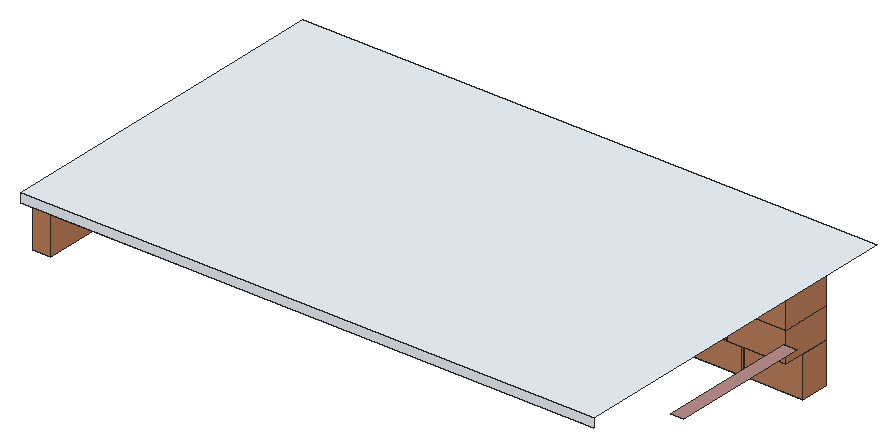
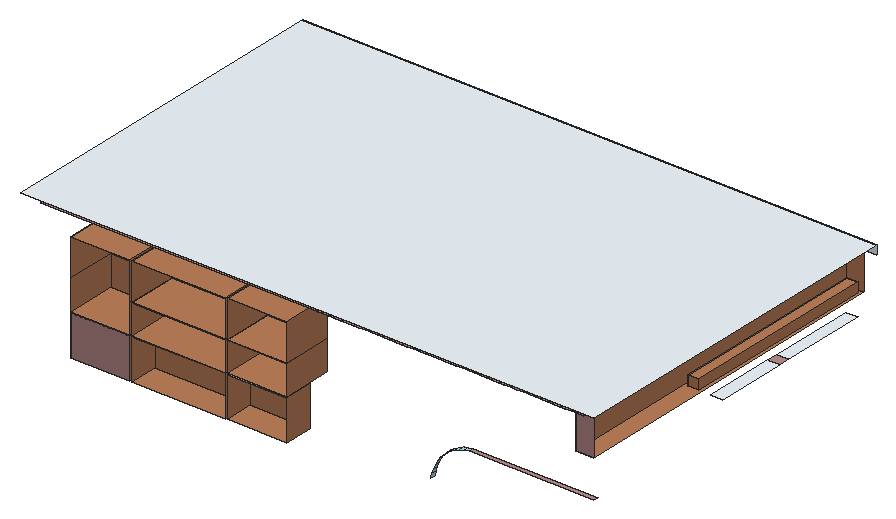
# SketchUp Ruby script. Lengths in inches.
U = 1.inch
M = Sketchup.active_model
def pt(a) = Geom::Point3d.new(a.map { |v| v * U })
def face(e, loops, mat)
  f = e.add_face(loops[0].map { |a| pt(a) })
  loops[1..].each { |l| e.add_face(l.map { |a| pt(a) }).erase! }
  f.material = f.back_material = mat if mat
  f
end
# faces: each face lists its corners as indices into pts; further lists are holes
def faces(e, pts, list, mat = nil) = list.each { |f| face(e, (f[0].is_a?(Array) ? f : [f]).map { |l| l.map { |i| pts[i] } }, mat) }
# xy, xz, yz: faces in a plane at the given z, y or x. An outline is a flat list of corners, or four numbers for a rectangle; further outlines are holes
def ring(l) = l.size == 4 ? [[l[0], l[1]], [l[2], l[1]], [l[2], l[3]], [l[0], l[3]]] : l.each_slice(2).to_a
def flat(e, list, mat, &to3) = list.each { |f| face(e, (f[0].is_a?(Array) ? f : [f]).map { |l| ring(l).map { |u, v| to3.(u, v) } }, mat) }
def xy(e, z, list, mat = nil) = flat(e, list, mat) { |x, y| [x, y, z] }
def xz(e, y, list, mat = nil) = flat(e, list, mat) { |x, z| [x, y, z] }
def yz(e, x, list, mat = nil) = flat(e, list, mat) { |y, z| [x, y, z] }
def lines(e, pts, list) = list.each { |a, b| e.add_line(pt(pts[a]), pt(pts[b])) }
# prism: a flat outline (further loops are holes) pulled along v
def prism(e, loops, v, mat = nil)
  f = face(e, loops, mat); d = Geom::Vector3d.new(v.map { |x| x * U })
  f.pushpull(f.normal.samedirection?(d) ? d.length : -d.length)
end
def box(e, o, s, mat = nil) = prism(e, [[o, [o[0] + s[0], o[1], o[2]], [o[0] + s[0], o[1] + s[1], o[2]], [o[0], o[1] + s[1], o[2]]]], [0, 0, s[2]], mat)
def at(x, y, z, deg = 0) = Geom::Transformation.translation(pt([x, y, z])) * Geom::Transformation.rotation(ORIGIN, Z_AXIS, deg.degrees)
def axes(o, x, y, z) = Geom::Transformation.new([*x, 0, *y, 0, *z, 0, *pt(o).to_a, 1])
def part(name) = M.definitions.add(name)
# library, detail: a bought-in or finely detailed component or shape, given as its bounding box
def library(name, o, s) = part(name).tap { |d| box(d.entities, o, s) }
def detail(e, o, s) = box(e.add_group.entities, o, s)
def put(e, d, t, mat = nil) = e.add_instance(d, t).tap { |i| i.material = mat if mat }
def group(e, t, mat = nil) = e.add_group.tap { |g| g.transformation = t; g.material = mat if mat }.entities
root = M.entities
M.materials.add("[0093_AliceBlue]").color = [240, 248, 255]
M.materials.add("[0095_LightBlue]").color = [173, 216, 230]
M.materials.add("[0119_RosyBrown]").color = [188, 143, 143]
M.materials.add("[Wood Veneer 02]").color = [190, 128, 91]
c1 = library("Group\#6",[-0.5,-0.5,0],[175.45,81.95,0.375])
xy(root,86.86,[[126.39,126.49,150.39,137.93],[151.09,126.49,188.68,137.93],[189.375,126.49,213.375,137.93]],"[Wood Veneer 02]")
xy(root,102.8,[[126.39,126.49,150.39,137.93]],"[0119_RosyBrown]")
xy(root,103.11,[[151.09,126.49,188.68,137.93],[189.375,126.49,213.375,137.93]],"[0119_RosyBrown]")
xy(root,103.42,[[126.39,117.86,150.39,137.93],[151.09,117.86,188.68,137.93],[189.375,117.86,213.375,137.93]],"[Wood Veneer 02]")
xy(root,107.93,[[4.97,133.77,55.03,135.55]],"[0119_RosyBrown]")
xy(root,115.3,[[126.39,117.86,150.39,137.93],[151.09,117.86,188.68,137.93]],"[Wood Veneer 02]")
xy(root,115.49,[[126.39,117.86,150.39,137.93],[151.09,117.86,188.68,137.93]],"[Wood Veneer 02]")
xy(root,119.86,[[0,9.26,4.95,43.72],[0,48.29,4.95,77.05]],"[0093_AliceBlue]")
xy(root,119.86,[[0,43.72,4.95,48.29]],"[0119_RosyBrown]")
xy(root,121.64,[[225.375,45.11,230.5,101.93]],"[0119_RosyBrown]")
xy(root,123.05,[[[4.95,0,12.13,135.55],[6.31,1.36,10.77,81.01]]],"[Wood Veneer 02]")
xy(root,126.8,[[6.31,1.36,10.77,81.01]],"[Wood Veneer 02]")
xy(root,130.36,[[126.39,117.86,150.39,137.93],[151.09,117.86,188.68,137.93],[189.375,117.86,213.375,137.93]],"[Wood Veneer 02]")
xy(root,138.36,[[12.13,0,225.125,5.1875],[12.13,5.1875,12.13,12.37,217.95,12.37,217.95,124.69,12.13,124.69,12.13,131.86,225.125,131.86,225.125,5.1875],[[12.13,12.37,217.95,124.69],[37.92,26.16,192.16,26.16,193.72,26.26,195.26,26.56,196.75,27.07,198.16,27.76,199.46,28.64,200.64,29.67,201.68,30.85,202.55,32.16,203.24,33.5625,203.75,35.05,204.05,36.59,204.16,38.16,204.16,98.89,204.05,100.46,203.75,102,203.24,103.49,202.55,104.89,201.68,106.2,200.64,107.38,199.46,108.42,198.16,109.29,196.75,109.98,195.26,110.49,193.72,110.79,192.16,110.89,37.92,110.89,36.35,110.79,34.8125,110.49,33.33,109.98,31.92,109.29,30.61,108.42,29.43,107.38,28.4,106.2,27.53,104.89,26.83,103.49,26.33,102,26.02,100.46,25.92,98.89,25.92,38.16,26.16,36.65,26.58,35.18,27.16,33.76,27.9,32.42,28.78,31.17,29.8,30.03,30.9375,29.02,32.18,28.13,33.52,27.4,34.9375,26.82,36.41,26.4]],[[38.07,28.05,36.82,28.26,35.56,28.61,34.34,29.11,33.19,29.74,32.12,30.5,31.14,31.375,30.26,32.36,29.51,33.43,28.87,34.58,28.375,35.8,28.02,37.06,27.8125,38.31,27.8125,98.89,27.9,100.21,28.16,101.51,28.58,102.76,29.17,103.95,29.9,105.05,30.77,106.04,31.77,106.91,32.87,107.65,34.05,108.23,35.3,108.66,36.6,108.91,37.92,109,192.16,109,193.48,108.91,194.77,108.66,196.02,108.23,197.21,107.65,198.31,106.91,199.3,106.04,200.17,105.05,200.91,103.95,201.49,102.76,201.92,101.51,202.18,100.21,202.26,98.89,202.26,38.16,202.18,36.84,201.92,35.54,201.49,34.29,200.91,33.1,200.17,32,199.3,31.01,198.31,30.14,197.21,29.4,196.02,28.82,194.77,28.4,193.48,28.14,192.16,28.05],[49.92,38.16,180.16,38.16,181.72,38.26,183.26,38.56,184.75,39.07,186.16,39.76,187.46,40.64,188.64,41.67,189.68,42.85,190.55,44.16,191.24,45.5625,191.75,47.05,192.05,48.59,192.16,50.16,192.16,86.89,192.05,88.46,191.75,90,191.24,91.49,190.55,92.89,189.68,94.2,188.64,95.38,187.46,96.42,186.16,97.29,184.75,97.98,183.26,98.49,181.72,98.79,180.16,98.89,49.92,98.89,48.35,98.79,46.8125,98.49,45.33,97.98,43.92,97.29,42.61,96.42,41.43,95.38,40.4,94.2,39.53,92.89,38.83,91.49,38.33,90,38.02,88.46,37.92,86.89,37.92,50.16,37.97,48.57,38.24,47.01,38.72,45.5,39.4,44.07,40.27,42.74,41.31,41.55,42.5,40.51,43.83,39.64,45.26,38.96,46.77,38.48,48.33,38.21]],[49.83,40.68,48.59,40.72,47.37,40.93,46.1875,41.31,45.07,41.84,44.03,42.52,43.1,43.34,42.28,44.27,41.6,45.31,41.07,46.43,40.7,47.61,40.49,48.83,40.44,50.07,40.44,86.89,40.53,88.13,40.77,89.35,41.17,90.52,41.71,91.63,42.4,92.66,43.22,93.59,44.15,94.41,45.18,95.1,46.29,95.65,47.47,96.04,48.68,96.29,49.92,96.37,180.16,96.37,181.39,96.29,182.61,96.04,183.78,95.65,184.89,95.1,185.92,94.41,186.85,93.59,187.67,92.66,188.36,91.63,188.91,90.52,189.31,89.35,189.55,88.13,189.63,86.89,189.63,50.16,189.55,48.92,189.31,47.7,188.91,46.53,188.36,45.42,187.67,44.39,186.85,43.46,185.92,42.64,184.89,41.95,183.78,41.4,182.61,41.01,181.39,40.76,180.16,40.68]],"[0093_AliceBlue]")
xy(root,138.36,[[225.125,0,225.125,131.86,12.13,131.86,12.13,135.55,11.89,135.55,11.89,137.93,14.71,137.93,14.71,135.55,16.77,135.55,16.77,137.93,19.59,137.93,19.59,135.55,21.65,135.55,21.65,137.93,24.47,137.93,24.47,135.55,26.53,135.55,26.53,137.93,29.35,137.93,29.35,135.55,31.42,135.55,31.42,137.93,34.23,137.93,34.23,135.55,36.3,135.55,36.3,137.93,39.11,137.93,39.11,135.55,41.18,135.55,41.18,137.93,43.99,137.93,43.99,135.55,46.06,135.55,46.06,137.93,48.875,137.93,48.875,135.55,50.9375,135.55,50.9375,137.93,53.76,137.93,53.76,135.55,55.82,135.55,55.82,137.93,58.64,137.93,58.64,135.55,60.7,135.55,60.7,137.93,63.52,137.93,63.52,135.55,65.58,135.55,65.58,137.93,68.4,137.93,68.4,135.55,70.46,135.55,70.46,137.93,73.28,137.93,73.28,135.55,75.34,135.55,75.34,137.93,78.16,137.93,78.16,135.55,80.22,135.55,80.22,137.93,83.04,137.93,83.04,135.55,85.1,135.55,85.1,137.93,87.92,137.93,87.92,135.55,89.98,135.55,89.98,137.93,92.8,137.93,92.8,135.55,94.86,135.55,94.86,137.93,97.68,137.93,97.68,135.55,99.74,135.55,99.74,137.93,102.5625,137.93,102.5625,135.55,104.625,135.55,104.625,137.93,107.44,137.93,107.44,135.55,109.51,135.55,109.51,137.93,112.32,137.93,112.32,135.55,114.39,135.55,114.39,137.93,225.375,137.93,225.375,0],[7.01,135.55,9.83,137.93],[9.83,135.55,11.89,137.93],[14.71,135.55,16.77,137.93],[19.59,135.55,21.65,137.93],
  [24.47,135.55,26.53,137.93],[29.35,135.55,31.42,137.93],[34.23,135.55,36.3,137.93],[39.11,135.55,41.18,137.93],[43.99,135.55,46.06,137.93],
  [48.875,135.55,50.9375,137.93],[53.76,135.55,55.82,137.93],[58.64,135.55,60.7,137.93],[63.52,135.55,65.58,137.93],[68.4,135.55,70.46,137.93],
  [73.28,135.55,75.34,137.93],[78.16,135.55,80.22,137.93],[83.04,135.55,85.1,137.93],[87.92,135.55,89.98,137.93],[92.8,135.55,94.86,137.93],
  [97.68,135.55,99.74,137.93],[102.5625,135.55,104.625,137.93],[107.44,135.55,109.51,137.93],[112.32,135.55,114.05,137.93],[114.05,135.55,114.39,137.93]],"[0119_RosyBrown]")
xy(root,138.92,[[[37.92,26.16,36.41,26.4,34.9375,26.82,33.52,27.4,32.18,28.13,30.9375,29.02,29.8,30.03,28.78,31.17,27.9,32.42,27.16,33.76,26.58,35.18,26.16,36.65,25.92,38.16,25.92,98.89,26.02,100.46,26.33,102,26.83,103.49,27.53,104.89,28.4,106.2,29.43,107.38,30.61,108.42,31.92,109.29,33.33,109.98,34.8125,110.49,36.35,110.79,37.92,110.89,192.16,110.89,193.72,110.79,195.26,110.49,196.75,109.98,198.16,109.29,199.46,108.42,200.64,107.38,201.68,106.2,202.55,104.89,203.24,103.49,203.75,102,204.05,100.46,204.16,98.89,204.16,38.16,204.05,36.59,203.75,35.05,203.24,33.5625,202.55,32.16,201.68,30.85,200.64,29.67,199.46,28.64,198.16,27.76,196.75,27.07,195.26,26.56,193.72,26.26,192.16,26.16],[38.07,28.05,192.16,28.05,193.48,28.14,194.77,28.4,196.02,28.82,197.21,29.4,198.31,30.14,199.3,31.01,200.17,32,200.91,33.1,201.49,34.29,201.92,35.54,202.18,36.84,202.26,38.16,202.26,98.89,202.18,100.21,201.92,101.51,201.49,102.76,200.91,103.95,200.17,105.05,199.3,106.04,198.31,106.91,197.21,107.65,196.02,108.23,194.77,108.66,193.48,108.91,192.16,109,37.92,109,36.6,108.91,35.3,108.66,34.05,108.23,32.87,107.65,31.77,106.91,30.77,106.04,29.9,105.05,29.17,103.95,28.58,102.76,28.16,101.51,27.9,100.21,27.8125,98.89,27.8125,38.31,28.02,37.06,28.375,35.8,28.87,34.58,29.51,33.43,30.26,32.36,31.14,31.375,32.12,30.5,33.19,29.74,34.34,29.11,35.56,28.61,36.82,28.26]]],"[0119_RosyBrown]")
xy(root,139.11,[[[49.92,38.16,48.33,38.21,46.77,38.48,45.26,38.96,43.83,39.64,42.5,40.51,41.31,41.55,40.27,42.74,39.4,44.07,38.72,45.5,38.24,47.01,37.97,48.57,37.92,50.16,37.92,86.89,38.02,88.46,38.33,90,38.83,91.49,39.53,92.89,40.4,94.2,41.43,95.38,42.61,96.42,43.92,97.29,45.33,97.98,46.8125,98.49,48.35,98.79,49.92,98.89,180.16,98.89,181.72,98.79,183.26,98.49,184.75,97.98,186.16,97.29,187.46,96.42,188.64,95.38,189.68,94.2,190.55,92.89,191.24,91.49,191.75,90,192.05,88.46,192.16,86.89,192.16,50.16,192.05,48.59,191.75,47.05,191.24,45.5625,190.55,44.16,189.68,42.85,188.64,41.67,187.46,40.64,186.16,39.76,184.75,39.07,183.26,38.56,181.72,38.26,180.16,38.16],[49.83,40.68,180.16,40.68,181.39,40.76,182.61,41.01,183.78,41.4,184.89,41.95,185.92,42.64,186.85,43.46,187.67,44.39,188.36,45.42,188.91,46.53,189.31,47.7,189.55,48.92,189.63,50.16,189.63,86.89,189.55,88.13,189.31,89.35,188.91,90.52,188.36,91.63,187.67,92.66,186.85,93.59,185.92,94.41,184.89,95.1,183.78,95.65,182.61,96.04,181.39,96.29,180.16,96.37,49.92,96.37,48.68,96.29,47.47,96.04,46.29,95.65,45.18,95.1,44.15,94.41,43.22,93.59,42.4,92.66,41.71,91.63,41.17,90.52,40.77,89.35,40.53,88.13,40.44,86.89,40.44,50.07,40.49,48.83,40.7,47.61,41.07,46.43,41.6,45.31,42.28,44.27,43.1,43.34,44.03,42.52,45.07,41.84,46.1875,41.31,47.37,40.93,48.59,40.72]]],"[0119_RosyBrown]")
xy(root,141.75,[[0,0,230.5,141.75]],"[0093_AliceBlue]")
xz(root,0,[[0,138.36,230.5,141.75]],"[0093_AliceBlue]")
xz(root,0,[[4.95,123.05,12.13,138.36]],"[Wood Veneer 02]")
xz(root,1.36,[[6.31,123.05,10.77,126.8]],"[Wood Veneer 02]")
xz(root,26.16,[[37.92,138.36,192.16,138.92]],"[0119_RosyBrown]")
xz(root,28.05,[[38.07,138.74,192.16,138.92]],"[0119_RosyBrown]")
xz(root,38.16,[[49.92,138.36,180.16,139.11]],"[0119_RosyBrown]")
xz(root,40.68,[[49.83,138.74,180.16,139.11]],"[0119_RosyBrown]")
xz(root,81.01,[[6.31,123.05,10.77,126.8]],"[Wood Veneer 02]")
xz(root,96.37,[[49.92,138.74,180.16,139.11]],"[0119_RosyBrown]")
xz(root,98.89,[[49.92,138.36,180.16,139.11]],"[0119_RosyBrown]")
xz(root,109,[[37.92,138.74,192.16,138.92]],"[0119_RosyBrown]")
xz(root,110.89,[[37.92,138.36,192.16,138.92]],"[0119_RosyBrown]")
xz(root,117.86,[[126.39,103.42,150.39,115.3],[151.09,103.42,188.68,115.3],[189.375,103.42,213.375,115.49],[126.39,115.49,150.39,130.36],[151.09,115.49,188.68,130.36],
  [189.375,115.49,213.375,130.36]],"[Wood Veneer 02]")
xz(root,126.49,[[126.39,86.86,150.39,102.8],[151.09,86.86,188.68,103.11],[189.375,86.86,213.375,103.11]],"[Wood Veneer 02]")
xz(root,135.55,[[4.95,123.05,12.13,138.36]],"[0119_RosyBrown]")
xz(root,137.93,[[189.375,86.86,213.375,103.11]],"[0119_RosyBrown]")
yz(root,6.31,[[1.36,123.05,81.01,126.8]],"[Wood Veneer 02]")
yz(root,10.77,[[1.36,123.05,81.01,126.8]],"[Wood Veneer 02]")
yz(root,12.13,[[0,123.05,135.55,138.36]],"[Wood Veneer 02]")
yz(root,25.92,[[38.16,138.36,98.89,138.92]],"[0119_RosyBrown]")
yz(root,27.8125,[[38.31,138.74,98.89,138.92]],"[0119_RosyBrown]")
yz(root,37.92,[[50.16,138.36,86.89,139.11]],"[0119_RosyBrown]")
yz(root,40.44,[[50.07,138.74,86.89,139.11]],"[0119_RosyBrown]")
yz(root,126.39,[[126.49,86.86,137.93,102.8],[117.86,103.42,137.93,115.3],[117.86,115.49,137.93,130.36]],"[Wood Veneer 02]")
yz(root,150.39,[[126.49,86.86,137.93,102.8],[117.86,103.42,137.93,115.3],[117.86,115.49,137.93,130.36]],"[Wood Veneer 02]")
yz(root,151.09,[[126.49,86.86,137.93,103.11],[117.86,103.42,137.93,115.3],[117.86,115.49,137.93,130.36]],"[Wood Veneer 02]")
yz(root,188.68,[[126.49,86.86,137.93,103.11],[117.86,103.42,137.93,115.3],[117.86,115.49,137.93,130.36]],"[Wood Veneer 02]")
yz(root,189.375,[[126.49,86.86,137.93,103.11],[117.86,103.42,137.93,115.49],[117.86,115.49,137.93,130.36]],"[Wood Veneer 02]")
yz(root,189.63,[[50.16,138.74,86.89,139.11]],"[0119_RosyBrown]")
yz(root,192.16,[[50.16,138.36,86.89,139.11]],"[0119_RosyBrown]")
yz(root,202.26,[[38.16,138.74,98.89,138.92]],"[0119_RosyBrown]")
yz(root,204.16,[[38.16,138.36,98.89,138.92]],"[0119_RosyBrown]")
yz(root,213.375,[[126.49,86.86,137.93,103.11],[117.86,103.42,137.93,115.49],[117.86,115.49,137.93,130.36]],"[Wood Veneer 02]")
p = [[70.01,135.55,94.53],[70.01,133.77,94.53],[70.35,133.77,92.61],[70.35,135.55,92.61],[69.47,135.55,96.4],[69.47,133.77,96.4],
  [68.71,135.55,98.19],[68.71,133.77,98.19],[67.77,135.55,99.89],[67.77,133.77,99.89],[66.64,135.55,101.48],[66.64,133.77,101.48],
  [65.34,135.55,102.93],[65.34,133.77,102.93],[63.89,135.55,104.22],[63.89,133.77,104.22],[62.31,135.55,105.35],[62.31,133.77,105.35],
  [60.61,135.55,106.3],[60.61,133.77,106.3],[58.8125,135.55,107.05],[58.8125,133.77,107.05],[56.95,135.55,107.6],[56.95,133.77,107.6],
  [55.03,135.55,107.93],[55.03,133.77,107.93],[37.92,26.16,138.36],[36.41,26.4,138.36],[36.41,26.4,138.92],[37.92,26.16,138.92],
  [193.72,26.26,138.36],[192.16,26.16,138.36],[192.16,26.16,138.92],[193.72,26.26,138.92],[195.26,26.56,138.36],[195.26,26.56,138.92],
  [34.9375,26.82,138.36],[34.9375,26.82,138.92],[196.75,27.07,138.36],[196.75,27.07,138.92],[33.52,27.4,138.36],[33.52,27.4,138.92],
  [198.16,27.76,138.36],[198.16,27.76,138.92],[32.18,28.13,138.36],[32.18,28.13,138.92],[199.46,28.64,138.36],[199.46,28.64,138.92],
  [30.9375,29.02,138.36],[30.9375,29.02,138.92],[200.64,29.67,138.36],[200.64,29.67,138.92],[29.8,30.03,138.36],[29.8,30.03,138.92],
  [201.68,30.85,138.36],[201.68,30.85,138.92],[28.78,31.17,138.36],[28.78,31.17,138.92],[202.55,32.16,138.36],[202.55,32.16,138.92],
  [27.9,32.42,138.36],[27.9,32.42,138.92],[203.24,33.5625,138.36],[203.24,33.5625,138.92],[27.16,33.76,138.36],[27.16,33.76,138.92],
  [203.75,35.05,138.36],[203.75,35.05,138.92],[26.58,35.18,138.36],[26.58,35.18,138.92],[204.05,36.59,138.36],[204.05,36.59,138.92],
  [26.16,36.65,138.36],[26.16,36.65,138.92],[25.92,38.16,138.36],[25.92,38.16,138.92],[204.16,38.16,138.36],[204.16,38.16,138.92],
  [48.33,38.21,138.36],[46.77,38.48,138.36],[46.77,38.48,139.11],[48.33,38.21,139.11],[49.92,38.16,138.36],[49.92,38.16,139.11],
  [181.72,38.26,138.36],[180.16,38.16,138.36],[180.16,38.16,139.11],[181.72,38.26,139.11],[183.26,38.56,138.36],[183.26,38.56,139.11],
  [45.26,38.96,138.36],[45.26,38.96,139.11],[184.75,39.07,138.36],[184.75,39.07,139.11],[43.83,39.64,138.36],[43.83,39.64,139.11],
  [186.16,39.76,138.36],[186.16,39.76,139.11],[42.5,40.51,138.36],[42.5,40.51,139.11],[187.46,40.64,138.36],[187.46,40.64,139.11],
  [41.31,41.55,138.36],[41.31,41.55,139.11],[188.64,41.67,138.36],[188.64,41.67,139.11],[40.27,42.74,138.36],[40.27,42.74,139.11],
  [189.68,42.85,138.36],[189.68,42.85,139.11],[39.4,44.07,138.36],[39.4,44.07,139.11],[190.55,44.16,138.36],[190.55,44.16,139.11],
  [38.72,45.5,138.36],[38.72,45.5,139.11],[191.24,45.5625,138.36],[191.24,45.5625,139.11],[38.24,47.01,138.36],[38.24,47.01,139.11],
  [191.75,47.05,138.36],[191.75,47.05,139.11],[37.97,48.57,138.36],[37.97,48.57,139.11],[192.05,48.59,138.36],[192.05,48.59,139.11],
  [37.92,50.16,138.36],[37.92,50.16,139.11],[192.16,50.16,138.36],[192.16,50.16,139.11],[37.92,86.89,138.36],[38.02,88.46,138.36],
  [38.02,88.46,139.11],[37.92,86.89,139.11],[192.05,88.46,138.36],[192.16,86.89,138.36],[192.16,86.89,139.11],[192.05,88.46,139.11],
  [38.33,90,138.36],[38.33,90,139.11],[191.75,90,138.36],[191.75,90,139.11],[38.83,91.49,138.36],[38.83,91.49,139.11],
  [191.24,91.49,138.36],[191.24,91.49,139.11],[39.53,92.89,138.36],[39.53,92.89,139.11],[190.55,92.89,138.36],[190.55,92.89,139.11],
  [40.4,94.2,138.36],[40.4,94.2,139.11],[189.68,94.2,138.36],[189.68,94.2,139.11],[41.43,95.38,138.36],[41.43,95.38,139.11],
  [188.64,95.38,138.36],[188.64,95.38,139.11],[42.61,96.42,138.36],[42.61,96.42,139.11],[187.46,96.42,138.36],[187.46,96.42,139.11],
  [43.92,97.29,138.36],[43.92,97.29,139.11],[186.16,97.29,138.36],[186.16,97.29,139.11],[45.33,97.98,138.36],[45.33,97.98,139.11],
  [184.75,97.98,138.36],[184.75,97.98,139.11],[46.8125,98.49,138.36],[46.8125,98.49,139.11],[183.26,98.49,138.36],[183.26,98.49,139.11],
  [48.35,98.79,138.36],[48.35,98.79,139.11],[181.72,98.79,138.36],[181.72,98.79,139.11],[49.92,98.89,138.36],[49.92,98.89,139.11],
  [180.16,98.89,138.36],[180.16,98.89,139.11],[25.92,98.89,138.36],[26.02,100.46,138.36],[26.02,100.46,138.92],[25.92,98.89,138.92],
  [27.8125,98.89,138.36],[27.8125,98.89,138.74],[27.9,100.21,138.74],[27.9,100.21,138.36],[204.05,100.46,138.36],[204.16,98.89,138.36],
  [204.16,98.89,138.92],[204.05,100.46,138.92],[28.16,101.51,138.74],[28.16,101.51,138.36],[26.33,102,138.36],[26.33,102,138.92],
  [203.75,102,138.36],[203.75,102,138.92],[28.58,102.76,138.74],[28.58,102.76,138.36],[26.83,103.49,138.36],[26.83,103.49,138.92],
  [203.24,103.49,138.36],[203.24,103.49,138.92],[29.17,103.95,138.74],[29.17,103.95,138.36],[27.53,104.89,138.36],[27.53,104.89,138.92],
  [202.55,104.89,138.36],[202.55,104.89,138.92],[29.9,105.05,138.74],[29.9,105.05,138.36],[28.4,106.2,138.36],[28.4,106.2,138.92],
  [201.68,106.2,138.36],[201.68,106.2,138.92],[30.77,106.04,138.74],[30.77,106.04,138.36],[31.77,106.91,138.74],[31.77,106.91,138.36],
  [29.43,107.38,138.36],[29.43,107.38,138.92],[200.64,107.38,138.36],[200.64,107.38,138.92],[32.87,107.65,138.74],[32.87,107.65,138.36],
  [30.61,108.42,138.36],[30.61,108.42,138.92],[199.46,108.42,138.36],[199.46,108.42,138.92],[34.05,108.23,138.74],[34.05,108.23,138.36],
  [35.3,108.66,138.74],[35.3,108.66,138.36],[31.92,109.29,138.36],[31.92,109.29,138.92],[198.16,109.29,138.36],[198.16,109.29,138.92],
  [36.6,108.91,138.74],[36.6,108.91,138.36],[37.92,109,138.74],[37.92,109,138.36],[33.33,109.98,138.36],[33.33,109.98,138.92],
  [196.75,109.98,138.36],[196.75,109.98,138.92],[34.8125,110.49,138.36],[34.8125,110.49,138.92],[195.26,110.49,138.36],[195.26,110.49,138.92],
  [36.35,110.79,138.36],[36.35,110.79,138.92],[193.72,110.79,138.36],[193.72,110.79,138.92],[37.92,110.89,138.36],[37.92,110.89,138.92],
  [192.16,110.89,138.36],[192.16,110.89,138.92],[36.82,28.26,138.92],[36.82,28.26,138.74],[38.07,28.05,138.74],[38.07,28.05,138.92],
  [192.16,28.05,138.92],[192.16,28.05,138.74],[193.48,28.14,138.74],[193.48,28.14,138.92],[194.77,28.4,138.74],[194.77,28.4,138.92],
  [35.56,28.61,138.92],[35.56,28.61,138.74],[196.02,28.82,138.74],[196.02,28.82,138.92],[34.34,29.11,138.92],[34.34,29.11,138.74],
  [197.21,29.4,138.74],[197.21,29.4,138.92],[33.19,29.74,138.92],[33.19,29.74,138.74],[198.31,30.14,138.74],[198.31,30.14,138.92],
  [32.12,30.5,138.92],[32.12,30.5,138.74],[199.3,31.01,138.74],[199.3,31.01,138.92],[31.14,31.375,138.92],[31.14,31.375,138.74],
  [200.17,32,138.74],[200.17,32,138.92],[30.26,32.36,138.92],[30.26,32.36,138.74],[200.91,33.1,138.74],[200.91,33.1,138.92],
  [29.51,33.43,138.92],[29.51,33.43,138.74],[201.49,34.29,138.74],[201.49,34.29,138.92],[28.87,34.58,138.92],[28.87,34.58,138.74],
  [201.92,35.54,138.74],[201.92,35.54,138.92],[28.375,35.8,138.92],[28.375,35.8,138.74],[202.18,36.84,138.74],[202.18,36.84,138.92],
  [28.02,37.06,138.92],[28.02,37.06,138.74],[202.26,38.16,138.74],[202.26,38.16,138.92],[27.8125,38.31,138.92],[27.8125,38.31,138.74],
  [47.37,40.93,139.11],[47.37,40.93,138.74],[48.59,40.72,138.74],[48.59,40.72,139.11],[49.83,40.68,138.74],[49.83,40.68,139.11],
  [180.16,40.68,139.11],[180.16,40.68,138.74],[181.39,40.76,138.74],[181.39,40.76,139.11],[182.61,41.01,138.74],[182.61,41.01,139.11],
  [46.1875,41.31,139.11],[46.1875,41.31,138.74],[183.78,41.4,138.74],[183.78,41.4,139.11],[45.07,41.84,139.11],[45.07,41.84,138.74],
  [184.89,41.95,138.74],[184.89,41.95,139.11],[44.03,42.52,139.11],[44.03,42.52,138.74],[185.92,42.64,138.74],[185.92,42.64,139.11],
  [43.1,43.34,139.11],[43.1,43.34,138.74],[186.85,43.46,138.74],[186.85,43.46,139.11],[42.28,44.27,139.11],[42.28,44.27,138.74],
  [187.67,44.39,138.74],[187.67,44.39,139.11],[41.6,45.31,139.11],[41.6,45.31,138.74],[188.36,45.42,138.74],[188.36,45.42,139.11],
  [41.07,46.43,139.11],[41.07,46.43,138.74],[188.91,46.53,138.74],[188.91,46.53,139.11],[40.7,47.61,139.11],[40.7,47.61,138.74],
  [189.31,47.7,138.74],[189.31,47.7,139.11],[40.49,48.83,139.11],[40.49,48.83,138.74],[189.55,48.92,138.74],[189.55,48.92,139.11],
  [40.44,50.07,139.11],[40.44,50.07,138.74],[189.63,50.16,138.74],[189.63,50.16,139.11],[40.53,88.13,139.11],[40.53,88.13,138.74],
  [40.44,86.89,138.74],[40.44,86.89,139.11],[189.63,86.89,139.11],[189.63,86.89,138.74],[189.55,88.13,138.74],[189.55,88.13,139.11],
  [40.77,89.35,139.11],[40.77,89.35,138.74],[189.31,89.35,138.74],[189.31,89.35,139.11],[41.17,90.52,139.11],[41.17,90.52,138.74],
  [188.91,90.52,138.74],[188.91,90.52,139.11],[41.71,91.63,139.11],[41.71,91.63,138.74],[188.36,91.63,138.74],[188.36,91.63,139.11],
  [42.4,92.66,139.11],[42.4,92.66,138.74],[187.67,92.66,138.74],[187.67,92.66,139.11],[43.22,93.59,139.11],[43.22,93.59,138.74],
  [186.85,93.59,138.74],[186.85,93.59,139.11],[44.15,94.41,139.11],[44.15,94.41,138.74],[185.92,94.41,138.74],[185.92,94.41,139.11],
  [45.18,95.1,139.11],[45.18,95.1,138.74],[184.89,95.1,138.74],[184.89,95.1,139.11],[46.29,95.65,139.11],[46.29,95.65,138.74],
  [183.78,95.65,138.74],[183.78,95.65,139.11],[47.47,96.04,139.11],[47.47,96.04,138.74],[182.61,96.04,138.74],[182.61,96.04,139.11],
  [48.68,96.29,139.11],[48.68,96.29,138.74],[181.39,96.29,138.74],[181.39,96.29,139.11],[49.92,96.37,139.11],[49.92,96.37,138.74],
  [180.16,96.37,138.74],[180.16,96.37,139.11],[27.9,100.21,138.92],[27.8125,98.89,138.92],[202.26,98.89,138.92],[202.26,98.89,138.74],
  [202.18,100.21,138.74],[202.18,100.21,138.92],[28.16,101.51,138.92],[201.92,101.51,138.74],[201.92,101.51,138.92],[28.58,102.76,138.92],
  [201.49,102.76,138.74],[201.49,102.76,138.92],[29.17,103.95,138.92],[200.91,103.95,138.74],[200.91,103.95,138.92],[29.9,105.05,138.92],
  [200.17,105.05,138.74],[200.17,105.05,138.92],[30.77,106.04,138.92],[199.3,106.04,138.74],[199.3,106.04,138.92],[31.77,106.91,138.92],
  [198.31,106.91,138.74],[198.31,106.91,138.92],[32.87,107.65,138.92],[197.21,107.65,138.74],[197.21,107.65,138.92],[34.05,108.23,138.92],
  [196.02,108.23,138.74],[196.02,108.23,138.92],[35.3,108.66,138.92],[194.77,108.66,138.74],[194.77,108.66,138.92],[36.6,108.91,138.92],
  [193.48,108.91,138.74],[193.48,108.91,138.92],[37.92,109,138.92],[192.16,109,138.74],[192.16,109,138.92],[0,137.93,138.36],
  [-0.3,137.93,138.36]]
faces(root,p,[[0,1,2,3],[4,5,1,0],[6,7,5,4],[8,9,7,6],[10,11,9,8],[12,13,11,10],[14,15,13,12],[16,17,15,14],
  [18,19,17,16],[20,21,19,18],[22,23,21,20],[24,25,23,22]],"[0095_LightBlue]")
faces(root,p,[[26,27,28,29],[30,31,32,33],[34,30,33,35],[27,36,37,28],[38,34,35,39],[36,40,41,37],[42,38,39,43],[40,44,45,41],
  [46,42,43,47],[44,48,49,45],[50,46,47,51],[48,52,53,49],[54,50,51,55],[52,56,57,53],[58,54,55,59],[56,60,61,57],
  [62,58,59,63],[60,64,65,61],[66,62,63,67],[64,68,69,65],[70,66,67,71],[68,72,73,69],[72,74,75,73],[76,70,71,77],
  [78,79,80,81],[82,78,81,83],[84,85,86,87],[88,84,87,89],[79,90,91,80],[92,88,89,93],[90,94,95,91],[96,92,93,97],
  [94,98,99,95],[100,96,97,101],[98,102,103,99],[104,100,101,105],[102,106,107,103],[108,104,105,109],[106,110,111,107],[112,108,109,113],
  [110,114,115,111],[116,112,113,117],[114,118,119,115],[120,116,117,121],[118,122,123,119],[124,120,121,125],[122,126,127,123],[128,124,125,129],
  [130,131,132,133],[134,135,136,137],[131,138,139,132],[140,134,137,141],[138,142,143,139],[144,140,141,145],[142,146,147,143],[148,144,145,149],
  [146,150,151,147],[152,148,149,153],[150,154,155,151],[156,152,153,157],[154,158,159,155],[160,156,157,161],[158,162,163,159],[164,160,161,165],
  [162,166,167,163],[168,164,165,169],[166,170,171,167],[172,168,169,173],[170,174,175,171],[176,172,173,177],[174,178,179,175],[180,176,177,181],
  [182,183,184,185],[186,187,188,189],[190,191,192,193],[189,188,194,195],[183,196,197,184],[198,190,193,199],[195,194,200,201],[196,202,203,197],
  [204,198,199,205],[201,200,206,207],[202,208,209,203],[210,204,205,211],[207,206,212,213],[208,214,215,209],[216,210,211,217],[213,212,218,219],
  [219,218,220,221],[214,222,223,215],[224,216,217,225],[221,220,226,227],[222,228,229,223],[230,224,225,231],[227,226,232,233],[233,232,234,235],
  [228,236,237,229],[238,230,231,239],[235,234,240,241],[241,240,242,243],[236,244,245,237],[246,238,239,247],[244,248,249,245],[250,246,247,251],
  [248,252,253,249],[254,250,251,255],[252,256,257,253],[258,254,255,259],[260,261,262,263],[264,265,266,267],[267,266,268,269],[270,271,261,260],
  [269,268,272,273],[274,275,271,270],[273,272,276,277],[278,279,275,274],[277,276,280,281],[282,283,279,278],[281,280,284,285],[286,287,283,282],
  [285,284,288,289],[290,291,287,286],[289,288,292,293],[294,295,291,290],[293,292,296,297],[298,299,295,294],[297,296,300,301],[302,303,299,298],
  [301,300,304,305],[306,307,303,302],[305,304,308,309],[310,311,307,306],[312,313,314,315],[315,314,316,317],[318,319,320,321],[321,320,322,323],
  [324,325,313,312],[323,322,326,327],[328,329,325,324],[327,326,330,331],[332,333,329,328],[331,330,334,335],[336,337,333,332],[335,334,338,339],
  [340,341,337,336],[339,338,342,343],[344,345,341,340],[343,342,346,347],[348,349,345,344],[347,346,350,351],[352,353,349,348],[351,350,354,355],
  [356,357,353,352],[355,354,358,359],[360,361,357,356],[359,358,362,363],[364,365,366,367],[368,369,370,371],[372,373,365,364],[371,370,374,375],
  [376,377,373,372],[375,374,378,379],[380,381,377,376],[379,378,382,383],[384,385,381,380],[383,382,386,387],[388,389,385,384],[387,386,390,391],
  [392,393,389,388],[391,390,394,395],[396,397,393,392],[395,394,398,399],[400,401,397,396],[399,398,402,403],[404,405,401,400],[403,402,406,407],
  [408,409,405,404],[407,406,410,411],[412,413,409,408],[411,410,414,415],[416,188,187,417],[418,419,420,421],[422,194,188,416],[421,420,423,424],
  [425,200,194,422],[424,423,426,427],[428,206,200,425],[427,426,429,430],[431,212,206,428],[430,429,432,433],[434,218,212,431],[433,432,435,436],
  [437,220,218,434],[436,435,438,439],[440,226,220,437],[439,438,441,442],[443,232,226,440],[442,441,444,445],[446,234,232,443],[445,444,447,448],
  [449,240,234,446],[448,447,450,451],[452,242,240,449],[451,450,453,454]],"[0119_RosyBrown]")
lines(root,p,[[455,456]])
put(root,c1,at(27.8125,28.05,138.36),"[0119_RosyBrown]")
